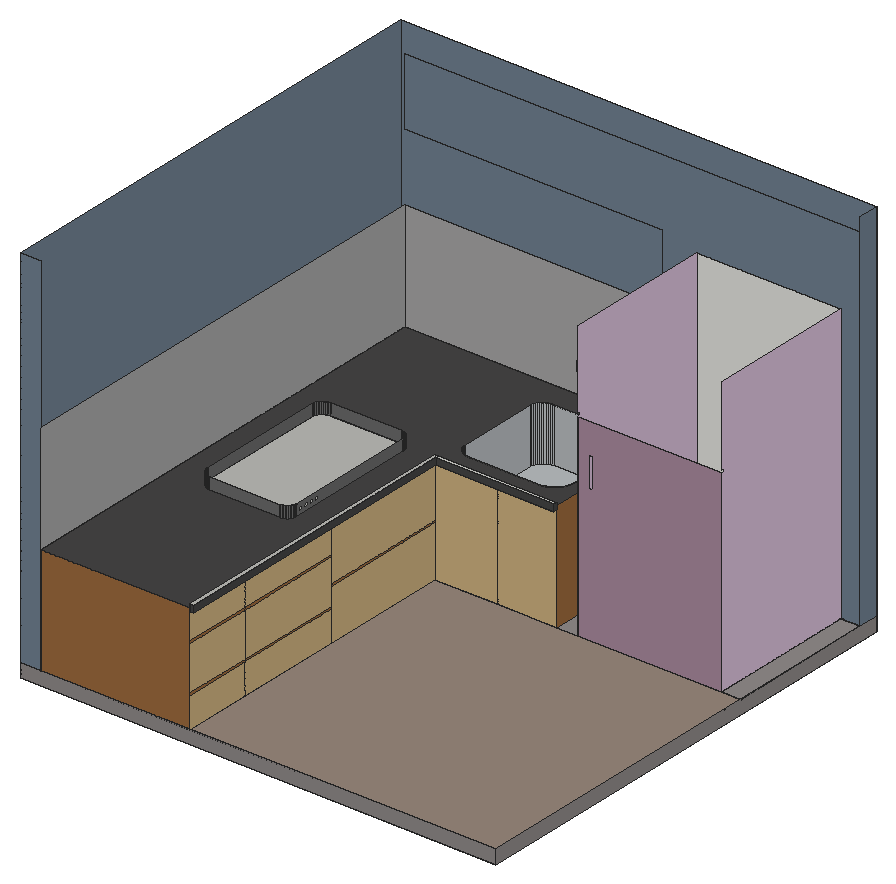
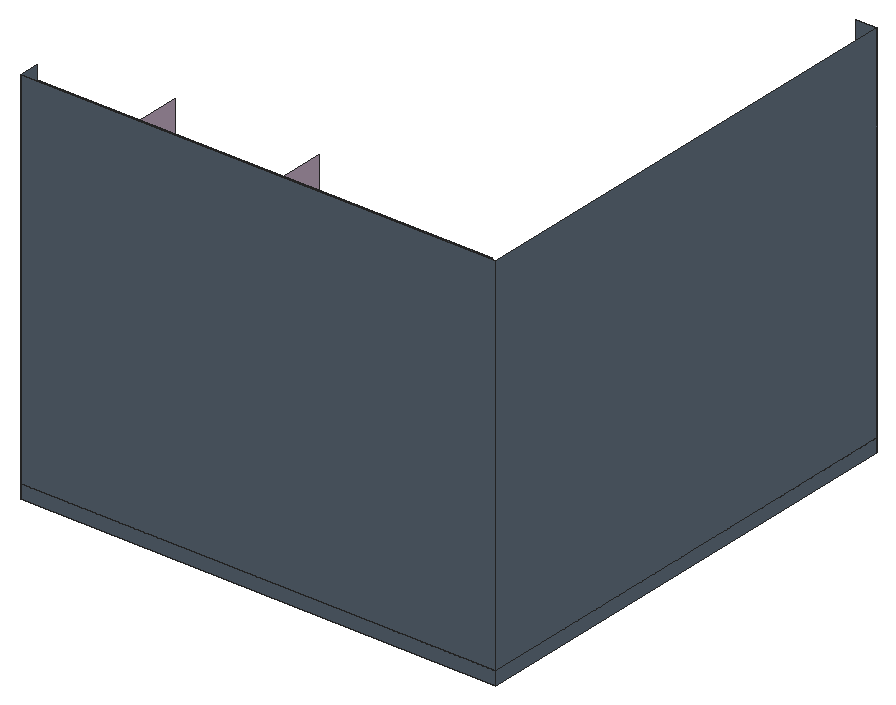
# SketchUp Ruby script. Lengths in inches.
U = 1.inch
M = Sketchup.active_model
def pt(a) = Geom::Point3d.new(a.map { |v| v * U })
def face(e, loops, mat)
  f = e.add_face(loops[0].map { |a| pt(a) })
  loops[1..].each { |l| e.add_face(l.map { |a| pt(a) }).erase! }
  f.material = f.back_material = mat if mat
  f
end
# faces: each face lists its corners as indices into pts; further lists are holes
def faces(e, pts, list, mat = nil) = list.each { |f| face(e, (f[0].is_a?(Array) ? f : [f]).map { |l| l.map { |i| pts[i] } }, mat) }
# xy, xz, yz: faces in a plane at the given z, y or x. An outline is a flat list of corners, or four numbers for a rectangle; further outlines are holes
def ring(l) = l.size == 4 ? [[l[0], l[1]], [l[2], l[1]], [l[2], l[3]], [l[0], l[3]]] : l.each_slice(2).to_a
def flat(e, list, mat, &to3) = list.each { |f| face(e, (f[0].is_a?(Array) ? f : [f]).map { |l| ring(l).map { |u, v| to3.(u, v) } }, mat) }
def xy(e, z, list, mat = nil) = flat(e, list, mat) { |x, y| [x, y, z] }
def xz(e, y, list, mat = nil) = flat(e, list, mat) { |x, z| [x, y, z] }
def yz(e, x, list, mat = nil) = flat(e, list, mat) { |y, z| [x, y, z] }
def lines(e, pts, list) = list.each { |a, b| e.add_line(pt(pts[a]), pt(pts[b])) }
# prism: a flat outline (further loops are holes) pulled along v
def prism(e, loops, v, mat = nil)
  f = face(e, loops, mat); d = Geom::Vector3d.new(v.map { |x| x * U })
  f.pushpull(f.normal.samedirection?(d) ? d.length : -d.length)
end
def box(e, o, s, mat = nil) = prism(e, [[o, [o[0] + s[0], o[1], o[2]], [o[0] + s[0], o[1] + s[1], o[2]], [o[0], o[1] + s[1], o[2]]]], [0, 0, s[2]], mat)
def at(x, y, z, deg = 0) = Geom::Transformation.translation(pt([x, y, z])) * Geom::Transformation.rotation(ORIGIN, Z_AXIS, deg.degrees)
def axes(o, x, y, z) = Geom::Transformation.new([*x, 0, *y, 0, *z, 0, *pt(o).to_a, 1])
def part(name) = M.definitions.add(name)
# library, detail: a bought-in or finely detailed component or shape, given as its bounding box
def library(name, o, s) = part(name).tap { |d| box(d.entities, o, s) }
def detail(e, o, s) = box(e.add_group.entities, o, s)
def put(e, d, t, mat = nil) = e.add_instance(d, t).tap { |i| i.material = mat if mat }
def group(e, t, mat = nil) = e.add_group.tap { |g| g.transformation = t; g.material = mat if mat }.entities
root = M.entities
M.materials.add("[0111_SlateGray]").color = [112, 128, 144]
M.materials.add("[0118_Thistle]").color = [216, 191, 216]
M.materials.add("[0134_DimGray]").color = [105, 105, 105]
M.materials.add("[Carpet Berber Multi]").color = [151, 134, 122]
M.materials.add("[Granite Dark Gray]").color = [69, 68, 68]
M.materials.add("[Plywood]").color = [168, 138, 158]
M.materials.add("[Steel Brushed Stainless]").color = [183, 187, 190]
M.materials.add("[Stone Marble]").color = [143, 138, 136]
M.materials.add("[Stone Vein Gray]").color = [166, 165, 165]
M.materials.add("[Wood Floor Light]").color = [204, 176, 127]
M.materials.add("[Wood Floor]").color = [155, 105, 61]
xy(root,0,[[0,0,420,420]])
xy(root,12,[[0,0,0,420,420,420,420,402,18,402,18,0],[18,0,18,402,228,402,228,270,150,270,150,0],[228,270,258,402],[276,270,403.2,402],[403.2,270,420,402]])
xy(root,12,[[150,0,420,270]],"[Carpet Berber Multi]")
xy(root,12,[[258,270,276,402]],"[Stone Marble]")
xy(root,12.03,[[403.2,270,420,402]],"[Stone Marble]")
xy(root,60,[[166.34,285.89,228.96,285.89,231.26,286.04,233.53,286.49,235.71,287.23,237.78,288.25,239.69,289.53,241.43,291.05,242.95,292.79,244.23,294.7,245.25,296.77,245.99,298.95,246.4375,301.21,246.59,303.51,246.59,368.53,246.49,370.05,246.19,371.54,245.7,372.97,245.03,374.34,244.1875,375.6,243.1875,376.74,242.05,377.74,240.78,378.59,239.42,379.26,237.98,379.74,236.49,380.04,234.98,380.14,166.7,380.14,165.18,380.04,163.69,379.74,162.26,379.26,160.89,378.59,159.63,377.74,158.49,376.74,157.49,375.6,156.64,374.34,155.97,372.97,155.48,371.54,155.1875,370.05,155.09,368.53,155.09,297.14,155.18,295.67,155.47,294.23,155.95,292.84,156.6,291.52,157.41,290.29,158.38,289.1875,159.49,288.22,160.71,287.4,162.03,286.75,163.43,286.27,164.87,285.99]],"[Steel Brushed Stainless]")
xy(root,105,[[150,0,150,270,258,270,258,267,153,267,153,0]],"[Granite Dark Gray]")
xy(root,108,[[[18,0,150,0,150,270,258,270,258,402,18,402],[56.8,138.66,55.54,138.74,54.3,138.99,53.11,139.39,51.98,139.95,50.93,140.65,49.98,141.48,49.15,142.43,48.45,143.48,47.9,144.61,47.49,145.8,47.25,147.04,47.16,148.29,47.16,262.65,47.25,263.91,47.49,265.14,47.9,266.34,48.45,267.47,49.15,268.51,49.98,269.46,50.93,270.29,51.98,270.99,53.11,271.55,54.3,271.96,55.54,272.2,56.8,272.28,118.35,272.28,119.44,272.21,120.52,272,121.55,271.65,122.54,271.16,123.45,270.55,124.27,269.83,124.99,269.01,125.6,268.1,126.09,267.11,126.44,266.08,126.65,265,126.73,263.91,126.73,147.04,126.65,145.94,126.44,144.87,126.09,143.83,125.6,142.85,124.99,141.9375,124.27,141.11,123.45,140.39,122.54,139.78,121.55,139.3,120.52,138.94,119.44,138.73,118.35,138.66],[166.34,285.89,164.87,285.99,163.43,286.27,162.03,286.75,160.71,287.4,159.49,288.22,158.38,289.1875,157.41,290.29,156.6,291.52,155.95,292.84,155.47,294.23,155.18,295.67,155.09,297.14,155.09,368.53,155.1875,370.05,155.48,371.54,155.97,372.97,156.64,374.34,157.49,375.6,158.49,376.74,159.63,377.74,160.89,378.59,162.26,379.26,163.69,379.74,165.18,380.04,166.7,380.14,234.98,380.14,236.49,380.04,237.98,379.74,239.42,379.26,240.78,378.59,242.05,377.74,243.1875,376.74,244.1875,375.6,245.03,374.34,245.7,372.97,246.19,371.54,246.49,370.05,246.59,368.53,246.59,303.51,246.4375,301.21,245.99,298.95,245.25,296.77,244.23,294.7,242.95,292.79,241.43,291.05,239.69,289.53,237.78,288.25,235.71,287.23,233.53,286.49,231.26,286.04,228.96,285.89]]],"[Granite Dark Gray]")
xz(root,0,[[0,12,18,336]],"[0111_SlateGray]")
xz(root,0,[[150,105,153,111]],"[Granite Dark Gray]")
xz(root,0,[[0,0,420,12]],"[Stone Marble]")
xz(root,0,[[18,12,150,108]],"[Wood Floor]")
xz(root,138.66,[[56.8,108,118.35,118]],"[0134_DimGray]")
xz(root,267,[[153,105,258,111]],"[Granite Dark Gray]")
xz(root,270,[[403.2,12,420,12.03],[150,105,153,108],[153,105,258,108],[150,108,153,111],[153,108,258,111]])
xz(root,270,[[[276,12,403.2,185.125],[286.47,131.625,289.54,158.25]]],"[Plywood]")
xz(root,270,[[150,12,205.71,105],[205.71,12,258,105]],"[Wood Floor Light]")
xz(root,272.28,[[56.8,108,118.35,118]],"[0134_DimGray]")
xz(root,285.89,[[166.34,60,228.96,108]],"[Steel Brushed Stainless]")
xz(root,380.14,[[166.7,60,234.98,108]],"[Steel Brushed Stainless]")
xz(root,402,[[18,12,228,108],[228,12,258,108],[276,12,403.2,257.125],[403.2,12,420,12.03]])
xz(root,402,[[403.2,12.03,420,12.03,420,324,18,324,18,264,245.68,264,245.68,204,276,204,276,257.125,403.2,257.125]],"[0111_SlateGray]")
xz(root,402,[[[258,12,276,12,276,204,18,204,18,108,258,108],[169.29,124.83,220.36,134.64]]],"[Stone Vein Gray]")
xz(root,420,[[0,0,420,12],[0,12,420,336]],"[0111_SlateGray]")
yz(root,0,[[0,0,420,12],[0,12,420,336]],"[0111_SlateGray]")
yz(root,18,[[0,12,402,108]])
yz(root,18,[[0,108,402,204]],"[Stone Vein Gray]")
yz(root,47.16,[[148.29,108,262.65,118]],"[0134_DimGray]")
yz(root,126.73,[[[147.04,108,263.91,118],[150.81,110.72,150.6,110.73,150.39,110.77,150.19,110.82,150,110.9,149.8125,111,149.64,111.11,149.48,111.25,149.33,111.4,149.2,111.5625,149.09,111.74,149,111.93,148.92,112.125,148.875,112.33,148.84,112.53,148.84,112.74,148.85,112.95,148.89,113.16,148.94,113.36,149.02,113.55,149.12,113.74,149.23,113.91,149.37,114.07,149.52,114.22,149.68,114.35,149.86,114.46,150.05,114.55,150.24,114.625,150.45,114.68,150.65,114.71,150.86,114.72,151.07,114.7,151.28,114.67,151.48,114.61,151.67,114.53,151.86,114.43,152.03,114.32,152.19,114.18,152.34,114.03,152.47,113.87,152.58,113.69,152.67,113.5,152.75,113.31,152.8,113.1,152.83,112.9,152.84,112.6875,152.82,112.48,152.79,112.27,152.73,112.07,152.65,111.875,152.55,111.69,152.4375,111.52,152.3,111.36,152.15,111.21,151.99,111.08,151.8125,110.97,151.625,110.875,151.43,110.8,151.22,110.75,151.02,110.72],[156.81,110.72,156.6,110.73,156.39,110.77,156.19,110.82,156,110.9,155.8125,111,155.64,111.11,155.48,111.25,155.33,111.4,155.2,111.5625,155.09,111.74,155,111.93,154.92,112.125,154.875,112.33,154.84,112.53,154.84,112.74,154.85,112.95,154.89,113.16,154.94,113.36,155.02,113.55,155.12,113.74,155.23,113.91,155.37,114.07,155.52,114.22,155.68,114.35,155.86,114.46,156.05,114.55,156.24,114.625,156.45,114.68,156.65,114.71,156.86,114.72,157.07,114.7,157.28,114.67,157.48,114.61,157.67,114.53,157.86,114.43,158.03,114.32,158.19,114.18,158.34,114.03,158.47,113.87,158.58,113.69,158.67,113.5,158.75,113.31,158.8,113.1,158.83,112.9,158.84,112.6875,158.82,112.48,158.79,112.27,158.73,112.07,158.65,111.875,158.55,111.69,158.4375,111.52,158.3,111.36,158.15,111.21,157.99,111.08,157.8125,110.97,157.625,110.875,157.43,110.8,157.22,110.75,157.02,110.72],[162.81,110.72,162.6,110.73,162.39,110.77,162.19,110.82,162,110.9,161.8125,111,161.64,111.11,161.48,111.25,161.33,111.4,161.2,111.5625,161.09,111.74,161,111.93,160.92,112.125,160.875,112.33,160.84,112.53,160.84,112.74,160.85,112.95,160.89,113.16,160.94,113.36,161.02,113.55,161.12,113.74,161.23,113.91,161.37,114.07,161.52,114.22,161.68,114.35,161.86,114.46,162.05,114.55,162.24,114.625,162.45,114.68,162.65,114.71,162.86,114.72,163.07,114.7,163.28,114.67,163.48,114.61,163.67,114.53,163.86,114.43,164.03,114.32,164.19,114.18,164.34,114.03,164.47,113.87,164.58,113.69,164.67,113.5,164.75,113.31,164.8,113.1,164.83,112.9,164.84,112.6875,164.82,112.48,164.79,112.27,164.73,112.07,164.65,111.875,164.55,111.69,164.4375,111.52,164.3,111.36,164.15,111.21,163.99,111.08,163.8125,110.97,163.625,110.875,163.43,110.8,163.22,110.75,163.02,110.72],[168.64,110.51,168.43,110.52,168.23,110.56,168.02,110.61,167.83,110.6875,167.64,110.79,167.47,110.9,167.31,111.03,167.16,111.18,167.03,111.34,166.91,111.52,166.82,111.71,166.75,111.9,166.69,112.11,166.66,112.3125,166.65,112.52,166.66,112.73,166.7,112.9375,166.75,113.14,166.83,113.33,166.92,113.52,167.04,113.7,167.17,113.86,167.32,114.01,167.48,114.14,167.66,114.25,167.85,114.34,168.04,114.42,168.25,114.47,168.45,114.5,168.66,114.51,168.87,114.5,169.08,114.47,169.28,114.41,169.47,114.34,169.66,114.24,169.84,114.125,170,113.99,170.14,113.84,170.28,113.68,170.39,113.5,170.48,113.32,170.56,113.12,170.61,112.92,170.64,112.71,170.65,112.5,170.64,112.29,170.61,112.09,170.55,111.89,170.47,111.69,170.38,111.5,170.26,111.33,170.13,111.17,169.98,111.02,169.82,110.89,169.64,110.78,169.46,110.68,169.26,110.61,169.06,110.55,168.85,110.52]]],"[0134_DimGray]")
yz(root,150,[[0,105,270,108],[0,108,270,111]])
yz(root,150,[[0,12,60,38.75],[60,12,156,38.75],[156,12,270,56.55],[0,40.75,60,79.75],[60,40.75,156,79.75],
  [156,58.5,270,105],[0,81.75,60,105],[60,81.75,156,105]],"[Wood Floor Light]")
yz(root,150,[[0,38.75,60,40.75],[60,38.75,156,40.75],[156,56.55,270,58.5],[0,79.75,60,81.75],[60,79.75,156,81.75]],"[Wood Floor]")
yz(root,153,[[0,105,267,111]],"[Granite Dark Gray]")
yz(root,155.09,[[297.14,60,368.53,108]],"[Steel Brushed Stainless]")
yz(root,246.59,[[303.51,60,368.53,108]],"[Steel Brushed Stainless]")
yz(root,258,[[267,105,270,111]],"[Granite Dark Gray]")
yz(root,258,[[270,12,402,108]],"[Wood Floor]")
yz(root,276,[[270,12,270,185.125,273,185.125,273,188.125,270,188.125,270,257.125,402,257.125,402,12]],"[0118_Thistle]")
yz(root,403.2,[[270,12,402,12.03]])
yz(root,403.2,[[270,12.03,402,12.03,402,257.125,270,257.125,270,188.125,273,188.125,273,185.125,270,185.125]],"[0118_Thistle]")
yz(root,420,[[270,12,402,12.03]])
yz(root,420,[[402,12,420,336]],"[0111_SlateGray]")
yz(root,420,[[0,0,420,12]],"[Stone Marble]")
p = [[164.87,285.99,108],[166.34,285.89,108],[166.34,285.89,60],[164.87,285.99,60],[228.96,285.89,108],[231.26,286.04,108],
  [231.26,286.04,60],[228.96,285.89,60],[163.43,286.27,108],[163.43,286.27,60],[233.53,286.49,108],[233.53,286.49,60],
  [162.03,286.75,108],[162.03,286.75,60],[235.71,287.23,108],[235.71,287.23,60],[160.71,287.4,108],[160.71,287.4,60],
  [237.78,288.25,108],[237.78,288.25,60],[159.49,288.22,108],[159.49,288.22,60],[158.38,289.1875,108],[158.38,289.1875,60],
  [239.69,289.53,108],[239.69,289.53,60],[157.41,290.29,108],[157.41,290.29,60],[241.43,291.05,108],[241.43,291.05,60],
  [156.6,291.52,108],[156.6,291.52,60],[242.95,292.79,108],[242.95,292.79,60],[155.95,292.84,108],[155.95,292.84,60],
  [155.47,294.23,108],[155.47,294.23,60],[244.23,294.7,108],[244.23,294.7,60],[155.18,295.67,108],[155.18,295.67,60],
  [245.25,296.77,108],[245.25,296.77,60],[155.09,297.14,108],[155.09,297.14,60],[245.99,298.95,108],[245.99,298.95,60],
  [246.4375,301.21,108],[246.4375,301.21,60],[246.59,303.51,108],[246.59,303.51,60],[155.1875,370.05,108],[155.09,368.53,108],
  [155.09,368.53,60],[155.1875,370.05,60],[246.59,368.53,108],[246.49,370.05,108],[246.49,370.05,60],[246.59,368.53,60],
  [155.48,371.54,108],[155.48,371.54,60],[246.19,371.54,108],[246.19,371.54,60],[155.97,372.97,108],[155.97,372.97,60],
  [245.7,372.97,108],[245.7,372.97,60],[156.64,374.34,108],[156.64,374.34,60],[245.03,374.34,108],[245.03,374.34,60],
  [157.49,375.6,108],[157.49,375.6,60],[244.1875,375.6,108],[244.1875,375.6,60],[158.49,376.74,108],[158.49,376.74,60],
  [243.1875,376.74,108],[243.1875,376.74,60],[159.63,377.74,108],[159.63,377.74,60],[242.05,377.74,108],[242.05,377.74,60],
  [160.89,378.59,108],[160.89,378.59,60],[240.78,378.59,108],[240.78,378.59,60],[162.26,379.26,108],[162.26,379.26,60],
  [239.42,379.26,108],[239.42,379.26,60],[163.69,379.74,108],[163.69,379.74,60],[237.98,379.74,108],[237.98,379.74,60],
  [165.18,380.04,108],[165.18,380.04,60],[236.49,380.04,108],[236.49,380.04,60],[166.7,380.14,108],[166.7,380.14,60],
  [234.98,380.14,108],[234.98,380.14,60],[54.3,138.99,108],[55.54,138.74,108],[55.54,138.74,118],[54.3,138.99,118],
  [56.8,138.66,108],[56.8,138.66,118],[118.35,138.66,108],[119.44,138.73,108],[119.44,138.73,118],[118.35,138.66,118],
  [120.52,138.94,108],[120.52,138.94,118],[121.55,139.3,108],[121.55,139.3,118],[53.11,139.39,108],[53.11,139.39,118],
  [122.54,139.78,108],[122.54,139.78,118],[51.98,139.95,108],[51.98,139.95,118],[123.45,140.39,108],[123.45,140.39,118],
  [50.93,140.65,108],[50.93,140.65,118],[124.27,141.11,108],[124.27,141.11,118],[49.98,141.48,108],[49.98,141.48,118],
  [124.99,141.9375,108],[124.99,141.9375,118],[49.15,142.43,108],[49.15,142.43,118],[125.6,142.85,108],[125.6,142.85,118],
  [48.45,143.48,108],[48.45,143.48,118],[126.09,143.83,108],[126.09,143.83,118],[47.9,144.61,108],[47.9,144.61,118],
  [126.44,144.87,108],[126.44,144.87,118],[47.49,145.8,108],[47.49,145.8,118],[126.65,145.94,108],[126.65,145.94,118],
  [47.25,147.04,108],[47.25,147.04,118],[126.73,147.04,108],[126.73,147.04,118],[47.16,148.29,108],[47.16,148.29,118],
  [47.25,263.91,108],[47.16,262.65,108],[47.16,262.65,118],[47.25,263.91,118],[47.49,265.14,108],[47.49,265.14,118],
  [126.73,263.91,108],[126.65,265,108],[126.65,265,118],[126.73,263.91,118],[126.44,266.08,108],[126.44,266.08,118],
  [47.9,266.34,108],[47.9,266.34,118],[126.09,267.11,108],[126.09,267.11,118],[48.45,267.47,108],[48.45,267.47,118],
  [125.6,268.1,108],[125.6,268.1,118],[49.15,268.51,108],[49.15,268.51,118],[124.99,269.01,108],[124.99,269.01,118],
  [49.98,269.46,108],[49.98,269.46,118],[124.27,269.83,108],[124.27,269.83,118],[50.93,270.29,108],[50.93,270.29,118],
  [123.45,270.55,108],[123.45,270.55,118],[51.98,270.99,108],[51.98,270.99,118],[122.54,271.16,108],[122.54,271.16,118],
  [53.11,271.55,108],[53.11,271.55,118],[121.55,271.65,108],[121.55,271.65,118],[54.3,271.96,108],[54.3,271.96,118],
  [120.52,272,108],[120.52,272,118],[55.54,272.2,108],[55.54,272.2,118],[119.44,272.21,108],[119.44,272.21,118],
  [56.8,272.28,108],[56.8,272.28,118],[118.35,272.28,108],[118.35,272.28,118]]
faces(root,p,[[0,1,2,3],[4,5,6,7],[8,0,3,9],[5,10,11,6],[12,8,9,13],[10,14,15,11],[16,12,13,17],[14,18,19,15],
  [20,16,17,21],[22,20,21,23],[18,24,25,19],[26,22,23,27],[24,28,29,25],[30,26,27,31],[28,32,33,29],[34,30,31,35],
  [36,34,35,37],[32,38,39,33],[40,36,37,41],[38,42,43,39],[44,40,41,45],[42,46,47,43],[46,48,49,47],[48,50,51,49],
  [52,53,54,55],[56,57,58,59],[60,52,55,61],[57,62,63,58],[64,60,61,65],[62,66,67,63],[68,64,65,69],[66,70,71,67],
  [72,68,69,73],[70,74,75,71],[76,72,73,77],[74,78,79,75],[80,76,77,81],[78,82,83,79],[84,80,81,85],[82,86,87,83],
  [88,84,85,89],[86,90,91,87],[92,88,89,93],[90,94,95,91],[96,92,93,97],[94,98,99,95],[100,96,97,101],[98,102,103,99]],"[Steel Brushed Stainless]")
faces(root,p,[[104,105,106,107],[105,108,109,106],[110,111,112,113],[111,114,115,112],[114,116,117,115],[118,104,107,119],[116,120,121,117],[122,118,119,123],
  [120,124,125,121],[126,122,123,127],[124,128,129,125],[130,126,127,131],[128,132,133,129],[134,130,131,135],[132,136,137,133],[138,134,135,139],
  [136,140,141,137],[142,138,139,143],[140,144,145,141],[146,142,143,147],[144,148,149,145],[150,146,147,151],[148,152,153,149],[154,150,151,155],
  [156,157,158,159],[160,156,159,161],[162,163,164,165],[163,166,167,164],[168,160,161,169],[166,170,171,167],[172,168,169,173],[170,174,175,171],
  [176,172,173,177],[174,178,179,175],[180,176,177,181],[178,182,183,179],[184,180,181,185],[182,186,187,183],[188,184,185,189],[186,190,191,187],
  [192,188,189,193],[190,194,195,191],[196,192,193,197],[194,198,199,195],[200,196,197,201],[198,202,203,199],[204,200,201,205],[202,206,207,203]],"[0134_DimGray]")
